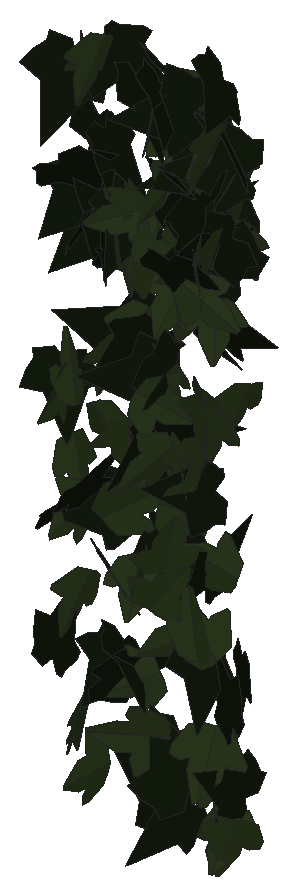
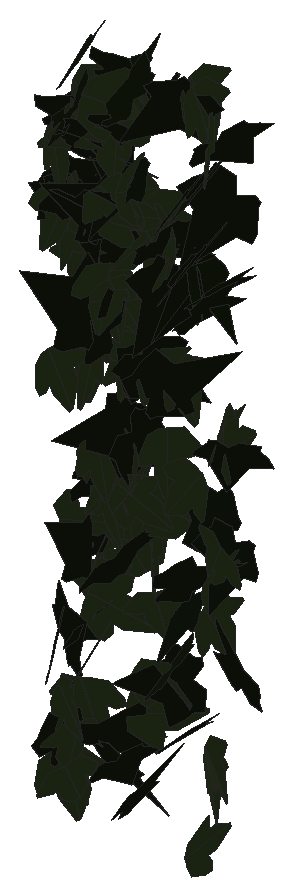
# SketchUp Ruby script. Lengths in inches.
U = 1.inch
M = Sketchup.active_model
def pt(a) = Geom::Point3d.new(a.map { |v| v * U })
def face(e, loops, mat)
  f = e.add_face(loops[0].map { |a| pt(a) })
  loops[1..].each { |l| e.add_face(l.map { |a| pt(a) }).erase! }
  f.material = f.back_material = mat if mat
  f
end
# faces: each face lists its corners as indices into pts; further lists are holes
def faces(e, pts, list, mat = nil) = list.each { |f| face(e, (f[0].is_a?(Array) ? f : [f]).map { |l| l.map { |i| pts[i] } }, mat) }
# xy, xz, yz: faces in a plane at the given z, y or x. An outline is a flat list of corners, or four numbers for a rectangle; further outlines are holes
def ring(l) = l.size == 4 ? [[l[0], l[1]], [l[2], l[1]], [l[2], l[3]], [l[0], l[3]]] : l.each_slice(2).to_a
def flat(e, list, mat, &to3) = list.each { |f| face(e, (f[0].is_a?(Array) ? f : [f]).map { |l| ring(l).map { |u, v| to3.(u, v) } }, mat) }
def xy(e, z, list, mat = nil) = flat(e, list, mat) { |x, y| [x, y, z] }
def xz(e, y, list, mat = nil) = flat(e, list, mat) { |x, z| [x, y, z] }
def yz(e, x, list, mat = nil) = flat(e, list, mat) { |y, z| [x, y, z] }
def lines(e, pts, list) = list.each { |a, b| e.add_line(pt(pts[a]), pt(pts[b])) }
# prism: a flat outline (further loops are holes) pulled along v
def prism(e, loops, v, mat = nil)
  f = face(e, loops, mat); d = Geom::Vector3d.new(v.map { |x| x * U })
  f.pushpull(f.normal.samedirection?(d) ? d.length : -d.length)
end
def box(e, o, s, mat = nil) = prism(e, [[o, [o[0] + s[0], o[1], o[2]], [o[0] + s[0], o[1] + s[1], o[2]], [o[0], o[1] + s[1], o[2]]]], [0, 0, s[2]], mat)
def at(x, y, z, deg = 0) = Geom::Transformation.translation(pt([x, y, z])) * Geom::Transformation.rotation(ORIGIN, Z_AXIS, deg.degrees)
def axes(o, x, y, z) = Geom::Transformation.new([*x, 0, *y, 0, *z, 0, *pt(o).to_a, 1])
def part(name) = M.definitions.add(name)
# library, detail: a bought-in or finely detailed component or shape, given as its bounding box
def library(name, o, s) = part(name).tap { |d| box(d.entities, o, s) }
def detail(e, o, s) = box(e.add_group.entities, o, s)
def put(e, d, t, mat = nil) = e.add_instance(d, t).tap { |i| i.material = mat if mat }
def group(e, t, mat = nil) = e.add_group.tap { |g| g.transformation = t; g.material = mat if mat }.entities
root = M.entities
M.materials.add("efeu1").color = [18, 25, 13]
M.materials.add("efeu2").color = [43, 57, 29]
c1 = part("ivyleaf_9")
p = [[1.54,2.16,1.25],[1.36,2.04,1.19],[-0.21,0.99,0.68],[-0.71,1.11,0.82],[-0.85,0.86,0.67],[-0.8,0.17,0.21],
  [-0.9,-0.01,0.1],[-0.67,-0.16,-0.02],[-0.08,-0.08,-0.05],[-0.03,-0.6,-0.4],[0.65,-0.88,-0.66],[0.83,-0.6,-0.49],
  [1.29,-0.42,-0.43],[1.8125,-0.07,-0.26],[1.21,0.44,0.15]]
faces(c1.entities,p,[[0,1,2,3,4,5,6,7,8,9,10,11,12,13,14]],"efeu1")
c2 = part("ivyleaf_10")
p = [[0,0.5,-0.03],[-0.0625,2.02,-0.43],[-0.19,2.01,-0.46],[-0.54,1.05,-0.29],[-0.52,0.625,-0.18],[-0.83,0.76,-0.28],
  [-1.16,0.64,-0.33],[-1.15,0.33,-0.24],[-0.77,-0.39,0.02],[-0.3,-0.51,0.16],[0.04,-0.48,0.23],[-0.02,2.01,-0.4375],
  [-0.06,2.01,-0.43],[0.04,-0.49,0.23],[0.67,-0.49,0.14],[1.38,0.36,-0.2],[1.375,0.51,-0.24],[0.81,0.65,-0.19],
  [0.62,0.59,-0.15],[0.6,1.09,-0.28],[0.5,1.23,-0.31]]
faces(c2.entities,p,[[0,1,2,3,4,5,6,7,8,9,10],[11,12,0,13,14,15,16,17,18,19,20]],"efeu2")
put(root,c1,axes([576.21,125.94,260.87],[-0.5506,-0.74533,-0.55036],[0.38765,0.39616,-0.92432],[0.84151,-0.67016,0.0657]))
put(root,c1,axes([576.47,127.02,268.23],[-0.57025,-0.7939,0.63016],[-0.06659,-0.69213,-0.93224],[1.01141,-0.49319,0.29391]))
put(root,c2,axes([575.95,126.82,256.61],[0.96253,-0.19997,0.66872],[0.6603,-0.1083,-0.98281],[0.22621,1.16701,0.02338]))
put(root,c2,axes([576.77,125.29,260.46],[-0.11829,0.29675,-1.12846],[-0.01256,-1.13451,-0.29702],[-1.16676,-0.01788,0.11761]))
put(root,c1,axes([576.81,125.82,274.53],[-0.50075,-1.11948,0.18316],[-0.05417,-0.17639,-1.22617],[1.13307,-0.50318,0.02233]))
put(root,c2,axes([576.83,126.14,254.72],[-0.36011,-0.16195,1.05103],[0.35145,-1.06543,-0.04376],[1.00368,0.31497,0.39242]))
put(root,c1,axes([577.15,124.5,255.5625],[0.24953,1.00718,0.30349],[0.07384,0.29437,-1.03763],[-1.04932,0.26023,-0.00085]))
put(root,c2,axes([577.32,124.98,260.53],[-0.17585,1.04846,-0.50782],[-0.19069,0.48074,1.05859],[1.14926,0.24019,0.09794]))
put(root,c1,axes([577.18,126.97,267.09],[-0.47197,-0.81281,0.70187],[-0.233,-0.6709,-0.93362],[1.04833,-0.51505,0.10849]))
put(root,c2,axes([577.1,126.91,242.76],[-0.13212,0.13974,1.10923],[0.30512,-1.07004,0.17114],[1.07556,0.32072,0.0877]))
put(root,c2,axes([577.24,125.83,274.95],[0.6333,-0.81491,-0.47969],[0.01212,0.58428,-0.97658],[0.94553,0.53831,0.33381]))
put(root,c1,axes([577.16,124.07,249.08],[-0.78556,0.63276,0.59494],[0.33945,-0.51471,0.99563],[0.79945,0.84032,0.16185]))
put(root,c2,axes([577.39,125.6875,246.19],[0.43696,-1.09032,-0.27127],[-0.06773,0.26497,-1.17411],[1.12152,0.44081,0.03479]))
put(root,c2,axes([577.38,125.61,246.37],[0.48178,-0.93781,0.23175],[0.08203,-0.21832,-1.054],[0.96253,0.48801,-0.02618]))
put(root,c1,axes([577.87,125.49,268.29],[-0.59633,0.87273,-0.40941],[0.26096,-0.3173,-1.05646],[-0.928,-0.65004,-0.03399]))
put(root,c1,axes([577.21,126.29,269.77],[0.70001,-0.81131,-0.51883],[-0.21487,0.49366,-1.06186],[0.93874,0.71798,0.14383]))
put(root,c1,axes([578.27,127.21,254.48],[-0.53873,-0.19896,0.96869],[-0.76645,-0.61306,-0.55217],[0.6249,-0.92345,0.15787]))
put(root,c1,axes([577.5,124.12,270.97],[0.86928,0.85438,0.20416],[0.14979,0.13884,-1.21885],[-0.86557,0.88207,-0.0059]))
put(root,c2,axes([577.95,124.9375,252.17],[-0.11238,-0.95158,0.57292],[0.10305,-0.58229,-0.94693],[1.10595,-0.04244,0.14645]))
put(root,c1,axes([577.8,127.3125,247.79],[-0.44821,-0.8113,0.54928],[0.03193,-0.6158,-0.8835],[0.97923,-0.35126,0.28022]))
put(root,c2,axes([578.1,125.54,275.79],[0.06295,-1.17056,0.18926],[0.02501,-0.18818,-1.17216],[1.1855,0.06612,0.01467]))
put(root,c1,axes([577.99,125.96,268.48],[0.41123,-0.47929,-0.98265],[-0.54866,0.81762,-0.62841],[0.94567,0.68279,0.06272]))
put(root,c2,axes([577.83,126.3,259.01],[-0.93039,0.27639,-0.58135],[0.54076,-0.21868,-0.9694],[-0.34919,-1.07507,0.04773]))
put(root,c1,axes([577.66,126.26,272.1],[0.29082,-1.10386,0.3311],[0.11974,-0.31068,-1.14098],[1.14621,0.31253,0.03519]))
put(root,c1,axes([577.87,124.38,256.04],[0.31681,1.1083,0.15053],[-0.05889,-0.13971,1.15255],[1.11692,-0.32172,0.01807]))
put(root,c1,axes([577.84,126.03,268.62],[-0.32755,0.05392,-1.11872],[1.10802,-0.15453,-0.33186],[-0.16348,-1.15539,-0.00782]))
put(root,c2,axes([578.52,125.1,276.04],[-0.10213,-1.01703,0.53635],[0.13712,-0.54539,-1.00807],[1.14159,-0.02548,0.16907]))
put(root,c1,axes([579.375,126.79,262.58],[-0.20051,-0.01144,1.31345],[-1.2324,-0.458,-0.19213],[0.45439,-1.24723,0.0585]))
put(root,c1,axes([578.47,125.47,253.2],[0.95814,-0.20517,-0.47825],[-0.45725,0.14656,-0.97893],[0.24849,1.06079,0.04275]))
put(root,c1,axes([578.29,126.03,271.8],[0.64655,-0.828,-0.4397],[-0.20014,0.39991,-1.04736],[0.91589,0.67189,0.08152]))
put(root,c2,axes([579.16,125.47,262.94],[-0.03901,-1.08579,0.28514],[-0.01642,-0.28473,-1.08647],[1.12248,-0.0419,-0.00598]))
put(root,c1,axes([578.48,125.7,275.86],[0.07251,-0.32705,-1.15112],[0.3601,1.10574,-0.29147],[1.14121,-0.32813,0.16511]))
put(root,c1,axes([579.18,125.57,267.0625],[0.86851,0.72592,0.00561],[0.00452,0.00335,-1.13194],[-0.72593,0.86852,-0.00033]))
put(root,c2,axes([579.44,126.58,263.64],[-0.31026,-0.8322,0.71685],[0.22495,-0.77725,-0.80496],[1.07509,-0.07753,0.3753]))
put(root,c2,axes([579.94,125.23,259.58],[-0.55275,-0.93491,-0.06473],[0.02577,0.05996,-1.08606],[0.93679,-0.55329,-0.00832]))
put(root,c1,axes([579.73,126.03,269.11],[-0.39487,-1.04404,0.26644],[-0.10896,-0.24363,-1.11612],[1.07198,-0.40934,-0.0153]))
put(root,c2,axes([579.73,126.08,252.9],[0.82819,0.62267,-0.15147],[-0.10524,-0.11201,-1.03583],[-0.63213,0.83445,-0.02601]))
put(root,c1,axes([579.43,124.44,248.64],[0.18496,0.71468,-0.82032],[0.04067,0.82697,0.72964],[1.08722,-0.15252,0.11226]))
put(root,c2,axes([579.73,125.16,267.96],[-0.33145,1.06439,-0.19666],[0.07101,-0.18385,-1.11473],[-1.08008,-0.33872,-0.01293]))
put(root,c2,axes([580.65,124.875,269.64],[0.49082,0.12753,-1.01683],[-1.01399,-0.10292,-0.50236],[-0.14849,1.1244,0.06935]))
put(root,c2,axes([579.43,125.78,269.24],[-0.43412,0.33455,-1.04055],[0.63954,-0.83021,-0.53374],[-0.88637,-0.76287,0.12453]))
put(root,c1,axes([580.44,125.99,263.6],[-0.00797,0.23814,-1.12079],[-0.23563,-1.0972,-0.23145],[-1.12132,0.22887,0.05661]))
put(root,c1,axes([579.39,125.67,249.65],[0.37757,-0.97928,0.3703],[0.21807,-0.31145,-1.046],[1.02399,0.42741,0.08622]))
put(root,c2,axes([580.82,125.46,248.77],[-0.51526,0.01279,0.89908],[-0.77336,-0.53494,-0.4356],[0.45872,-0.88751,0.27551]))
put(root,c2,axes([580.95,126.46,257.42],[-0.53989,-0.21117,0.91697],[-0.75089,-0.54043,-0.56656],[0.56708,-0.91665,0.12279]))
put(root,c2,axes([579.87,124.58,256.0625],[-0.35907,-0.57703,0.9887],[0.60638,0.78302,0.67721],[-0.97098,0.70238,0.0573]))
put(root,c2,axes([581.5,124.76,246.65],[-0.03433,0.03688,-1.24408],[-1.16134,-0.44855,0.01875],[-0.44762,1.16091,0.04677]))
put(root,c1,axes([580.16,125.61,274.89],[0.5095,-1.08808,0.14521],[0.06096,-0.1318,-1.20146],[1.09603,0.51313,-0.00068]))
put(root,c1,axes([580.32,126.27,258.43],[0.54738,-0.96438,-0.08653],[-0.02429,0.08569,-1.1087],[0.96795,0.54752,0.02111]))
put(root,c1,axes([581.62,125.1,262.38],[-0.58183,-0.11902,0.95034],[-0.91763,-0.24926,-0.59302],[0.27436,-1.08607,0.03196]))
put(root,c1,axes([581.26,126.06,243.02],[-0.08123,-1.19786,0.09461],[0.00875,0.09423,1.20061],[-1.20156,0.08167,0.00235]))
put(root,c1,axes([581.12,125.85,259.83],[-0.24908,0.25077,-1.09909],[0.39335,-1.03553,-0.32541],[-1.05649,-0.44467,0.13797]))
put(root,c2,axes([581.08,124.66,254.53],[0.46767,-0.92506,-0.4502],[-0.07729,0.46154,-1.02866],[1.02588,0.45648,0.12773]))
put(root,c1,axes([580.99,127,245.58],[-0.26876,-0.98309,0.00849],[0.00459,-0.01006,-1.01914],[0.98312,-0.26871,0.00708]))
put(root,c2,axes([582.07,126.06,269.46],[-0.04295,0.00128,1.14451],[-0.78021,-0.83799,-0.02834],[0.83737,-0.78073,0.0323]))
put(root,c2,axes([581.49,125.23,258.97],[0.00698,-0.3992,1.07691],[0.04751,-1.07591,-0.39914],[1.14754,0.04697,0.00997]))
put(root,c2,axes([581.35,124.28,268.01],[0.12351,-0.31709,-1.15718],[0.349,1.12249,-0.27033],[1.14796,-0.30714,0.20669]))
put(root,c2,axes([581.37,125.97,270.68],[0.06648,-0.35323,1.09107],[0.34784,-1.03521,-0.35634],[1.09281,0.35099,0.04704]))
put(root,c2,axes([581.85,126.18,266.12],[-0.81248,-0.56729,0.53644],[-0.12519,-0.66952,-0.89765],[0.77066,-0.70684,0.41973]))
put(root,c1,axes([580.77,126.4375,275.375],[0.45765,-0.77691,0.66757],[0.5377,-0.44012,-0.88083],[0.87185,0.67925,0.19282]))
put(root,c2,axes([581.7,125.26,263.2],[-1.05284,0.38551,-0.00447],[0.00223,-0.00691,-1.12119],[-0.38553,-1.05282,0.00572]))
put(root,c2,axes([581.99,126.42,270.65],[0.61709,0.63757,-0.66256],[-0.60665,-0.31734,-0.87038],[-0.691,0.84799,0.17244]))
put(root,c2,axes([581.29,125.97,258.97],[-0.68982,0.44031,-0.73253],[0.52781,-0.52093,-0.81016],[-0.67222,-0.86085,0.11558]))
put(root,c2,axes([581.36,125.2,273.91],[-0.00786,-0.67562,-0.94712],[0.29936,-0.91643,0.65124],[-1.12423,-0.2393,0.18003]))
put(root,c1,axes([581.36,126.73,254.51],[-0.01403,-1.35925,0.1072],[-0.00638,-0.10714,-1.35931],[1.36346,-0.01449,-0.00526]))
put(root,c2,axes([582.37,126.59,274.74],[-0.20083,-0.48441,1.10209],[-0.51328,-0.97622,-0.52262],[1.08895,-0.54948,-0.04309]))
put(root,c2,axes([582.25,126.15,256.72],[-0.95442,0.28591,0.35961],[-0.42452,-0.23189,-0.94233],[-0.17563,-0.99321,0.32353]))
put(root,c1,axes([582.63,124.08,263.47],[-0.73687,0.65635,0.50313],[-0.35817,0.35411,-0.98652],[-0.74541,-0.81897,-0.02333]))
put(root,c1,axes([581.36,125.47,259.82],[0.15555,0.57908,-0.98023],[0.24648,0.94874,0.59959],[1.1115,-0.29143,0.00421]))
put(root,c2,axes([581.79,126,273.28],[0.70511,1.00023,0.05462],[0.03197,0.04428,-1.22378],[-1.00121,0.70584,-0.00062]))
put(root,c1,axes([581.78,125.23,271.53],[1.12307,0.05674,-0.42471],[-0.42676,0.04132,-1.12297],[-0.03841,1.19998,0.05875]))
put(root,c2,axes([582.16,126.22,266.64],[-0.90994,-0.65821,-0.11627],[0.09201,0.07119,-1.12304],[0.66204,-0.91457,-0.00374]))
put(root,c2,axes([582.59,125.81,266],[-1.03367,-0.04626,0.44618],[-0.43596,-0.16035,-1.0266],[0.10564,-1.11438,0.12919]))
put(root,c2,axes([582.34,126.55,259.09],[-0.33517,-1.0338,0.07616],[-0.02345,-0.07246,-1.08677],[1.03633,-0.33599,0.00004]))
put(root,c1,axes([581.73,125.11,275.23],[0.17635,-0.89983,0.73727],[0.20436,-0.71014,-0.91559],[1.1452,0.26529,0.04986]))
put(root,c2,axes([582.99,125.54,251.45],[-0.36468,-0.36654,1.07429],[-0.75256,-0.76666,-0.51704],[0.84977,-0.83626,0.00314]))
put(root,c1,axes([583.36,124.75,275],[-0.97625,0.19992,0.70832],[-0.69045,0.15872,-0.99642],[-0.25489,-1.19566,-0.01384]))
put(root,c1,axes([582.12,126.13,251.04],[0.72563,-0.62599,-0.58774],[-0.40554,0.42843,-0.95699],[0.75686,0.82972,0.05071]))
put(root,c2,axes([582.36,124.58,254.77],[-0.67215,-0.88861,0.0708],[0.04706,0.05318,1.11418],[-0.89019,0.67378,0.00544]))
put(root,c1,axes([582.59,126.86,273.71],[-0.93178,-0.60027,-0.16865],[0.1233,0.11987,-1.10789],[0.6112,-0.93931,-0.03361]))
put(root,c2,axes([582.16,124.2,253.08],[-0.77828,-0.54053,0.59136],[0.47692,0.3499,0.94748],[-0.64376,0.91269,-0.01301]))
put(root,c1,axes([583.1,124.86,244.83],[-1.04588,-0.62987,0.12428],[0.11224,0.05451,1.22085],[-0.63213,1.05183,0.01115]))
put(root,c2,axes([582.24,123.57,262.4],[0.33226,0.53253,0.91579],[0.25829,0.89009,-0.6113],[-1.0274,0.39599,0.14248]))
put(root,c2,axes([582.47,124.73,257.16],[0.18422,0.48753,0.98825],[-0.02944,1.00379,-0.48971],[-1.10158,0.0547,0.17836]))
put(root,c1,axes([583.27,124.77,244.18],[-1.23884,0.12455,-0.04238],[0.04202,-0.00572,-1.24508],[-0.12467,-1.23955,0.00149]))
put(root,c2,axes([582.8,126.55,259.13],[0.15017,-0.99933,0.54967],[0.14507,-0.53318,-1.00898],[1.13127,0.20103,0.05642]))
put(root,c1,axes([581.93,126.5,264.51],[0.70764,-0.49837,0.69339],[0.55035,-0.42238,-0.86524],[0.6529,0.89618,-0.0222]))
put(root,c1,axes([583.12,126.4375,257.375],[-0.05185,-0.87247,-0.6914],[0.09733,-0.69305,0.86725],[-1.10895,-0.02003,0.10844]))
put(root,c1,axes([582.29,125.74,269.25],[0.06089,-0.01892,1.14687],[1.08231,0.38125,-0.05117],[-0.37982,1.08335,0.03804]))
put(root,c1,axes([583.9,126.28,272.18],[-1.12045,0.17029,0.52833],[-0.55134,-0.20323,-1.10375],[-0.06445,-1.22198,0.25719]))
put(root,c1,axes([583.17,123.84,268.7],[0.97347,0.50571,-0.51933],[-0.46547,-0.23049,-1.09695],[-0.55568,1.079,0.00908]))
put(root,c1,axes([583.14,126.92,270.16],[-0.84659,-0.84936,-0.4738],[0.34488,0.32516,-1.19915],[0.90937,-0.91404,0.01368]))
put(root,c1,axes([584.38,124.34,271.33],[-0.80544,0.95553,0.56764],[-0.3695,0.43094,-1.2497],[-1.0482,-0.88614,0.00435]))
put(root,c1,axes([583.4,125.8,253.57],[0.00101,-0.25126,1.08423],[0.6872,0.853,0.19704],[-0.87547,0.66928,0.15592]))
put(root,c2,axes([584.24,124.83,251.55],[0.75319,0.28695,0.9196],[-0.86877,-0.30202,0.8058],[0.41622,-1.14967,0.01784]))
put(root,c2,axes([583.79,125.25,262.25],[-1.04325,0.50035,0.09585],[-0.08694,0.04039,-1.15703],[-0.50197,-1.04687,0.00118]))
put(root,c1,axes([583.42,125.66,250.46],[-0.05858,-1.09476,0.14406],[-0.01449,-0.14349,-1.09631],[1.1041,-0.05997,-0.00675]))
put(root,c2,axes([584.46,125.69,254.62],[0.2853,0.10337,1.03599],[-0.97334,-0.35481,0.30345],[0.36956,-1.01429,-0.00057]))
put(root,c2,axes([584.47,123.88,268.96],[-0.02465,0.1348,1.21745],[-0.99898,0.70242,-0.09801],[-0.70879,-0.99469,0.09578]))
put(root,c1,axes([582.75,126.74,264.88],[0.5646,-0.40053,1.21788],[0.97576,-0.72893,-0.69208],[0.83159,1.12724,-0.0148]))
put(root,c2,axes([584.65,126.01,246.8125],[-0.41116,0.08311,0.95506],[-0.92929,0.22077,-0.41927],[-0.23554,-1.0161,-0.01298]))
put(root,c2,axes([584.36,123.73,252.19],[-0.01592,1.10423,-0.61306],[-0.28411,0.59426,1.07776],[1.23063,0.15148,0.24088]))
put(root,c2,axes([584.04,126.17,268.22],[-0.14593,0.73905,-0.88205],[-0.15392,-0.89366,-0.72332],[-1.1404,0.02605,0.21049]))
put(root,c2,axes([583.97,125.26,247.06],[1.20964,0.32086,-0.1164],[-0.10612,-0.05384,-1.25123],[-0.32441,1.21403,-0.02472]))
put(root,c1,axes([583.7,126.36,275.81],[-0.01247,-0.83516,0.7987],[0.06572,-0.79797,-0.83336],[1.15373,0.03643,0.0561]))
put(root,c1,axes([584.48,125.16,269.57],[0.20375,0.95345,-0.60198],[-0.08937,-0.59615,-0.97446],[-1.12403,0.22023,-0.03164]))
put(root,c2,axes([584.2,125.25,274.01],[0.25856,-0.98732,0.57844],[0.11483,-0.56764,-1.02021],[1.13851,0.28148,-0.02846]))
put(root,c1,axes([585,125.14,269.82],[-0.0298,-0.03397,-1.17134],[-0.83133,-0.82519,0.04508],[-0.82588,0.83186,-0.00312]))
put(root,c2,axes([583.79,125.17,272.85],[-0.14709,-0.36555,-1.08993],[0.72596,0.82246,-0.37382],[0.89138,-0.73016,0.1246]))
put(root,c2,axes([584.1,125.74,245.3],[0.35176,0.99388,0.12021],[0.03067,0.11666,-1.05425],[-1.00066,0.35296,0.00995]))
put(root,c2,axes([584.64,124.35,262.18],[-1.1752,0.0244,0.28981],[-0.29002,-0.00769,-1.17537],[-0.02185,-1.21038,0.01331]))
put(root,c2,axes([584.38,125.32,269.53],[0.25932,-1.16142,0.20107],[0.03422,-0.19838,-1.18998],[1.1782,0.26139,-0.00969]))
put(root,c1,axes([585.3125,125.59,272.65],[-0.81182,0.1497,0.86162],[-0.86836,0.00139,-0.81841],[-0.10368,-1.18382,0.108]))
put(root,c1,axes([583.69,126.61,273.74],[0.45477,-0.87993,0.56614],[0.24892,-0.5086,-0.99044],[1.01628,0.51833,-0.01075]))
put(root,c2,axes([584.28,126.41,269.42],[-1.09292,0.09392,-0.25663],[0.25688,-0.00789,-1.09687],[-0.09324,-1.12262,-0.01376]))
put(root,c2,axes([584.58,126.5625,262.16],[-0.23232,-1.01093,0.29277],[-0.07874,-0.28228,-1.0372],[1.04952,-0.24495,-0.01301]))
put(root,c2,axes([584.38,125.92,243.39],[0.53256,0.8297,-0.40362],[-0.20251,-0.34956,-0.98577],[-0.90017,0.56951,-0.01702]))
put(root,c1,axes([585.37,125.125,268.37],[-0.1865,0.18849,1.18471],[-1.15263,0.30408,-0.22983],[-0.33242,-1.16011,0.13225]))
put(root,c2,axes([584.22,125.06,266.48],[1.05763,0.28651,0.17736],[0.16544,0.06746,-1.09553],[-0.29355,1.07027,0.02158]))
put(root,c1,axes([584.81,126.28,244.5],[0.01258,0.09563,1.02364],[-0.7378,-0.7121,0.07559],[0.71599,-0.73547,0.05991]))
put(root,c2,axes([583.93,124.39,267.4],[-0.60345,-0.21094,-0.91125],[0.93512,-0.11218,-0.59329],[0.02059,-1.08717,0.23802]))
put(root,c1,axes([584.07,127.11,249.91],[0.13497,-0.03499,-1.0255],[0.92476,-0.44405,0.13686],[-0.44463,-0.93418,-0.02665]))
put(root,c2,axes([584.95,125.45,243.4],[-0.79536,-0.79375,0.31995],[-0.22157,-0.23092,-1.12365],[0.82663,-0.82562,0.00667]))
put(root,c2,axes([584.78,126.22,272.05],[0.15836,-1.1301,-0.14598],[-0.00557,0.14661,-1.14105],[1.13948,0.15778,0.01471]))
put(root,c1,axes([585.38,124.8,248.64],[0.08582,-0.13634,1.29108],[-0.49948,1.19083,0.15896],[-1.19832,-0.50612,0.0262]))
